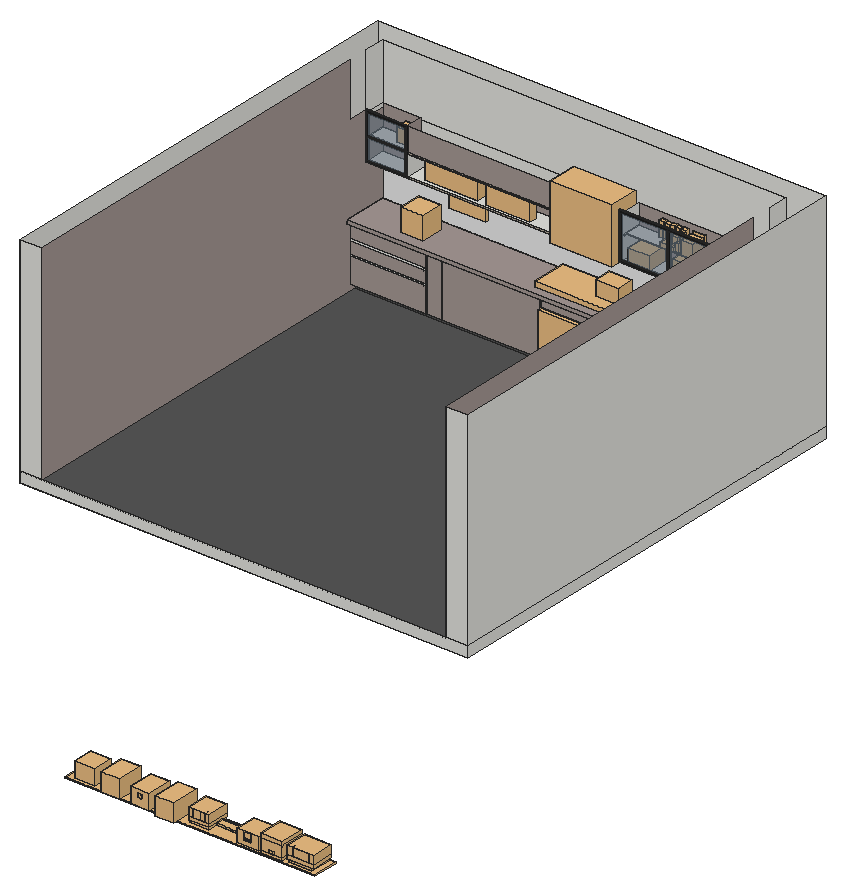
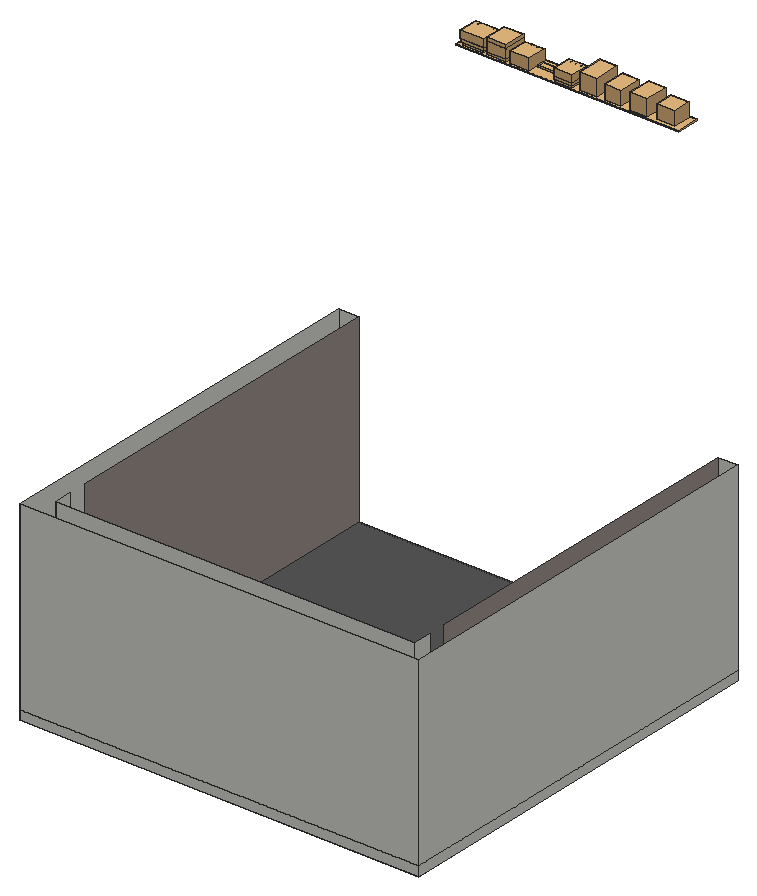
# SketchUp Ruby script. Lengths in inches.
U = 1.inch
M = Sketchup.active_model
def pt(a) = Geom::Point3d.new(a.map { |v| v * U })
def face(e, loops, mat)
  f = e.add_face(loops[0].map { |a| pt(a) })
  loops[1..].each { |l| e.add_face(l.map { |a| pt(a) }).erase! }
  f.material = f.back_material = mat if mat
  f
end
# faces: each face lists its corners as indices into pts; further lists are holes
def faces(e, pts, list, mat = nil) = list.each { |f| face(e, (f[0].is_a?(Array) ? f : [f]).map { |l| l.map { |i| pts[i] } }, mat) }
# xy, xz, yz: faces in a plane at the given z, y or x. An outline is a flat list of corners, or four numbers for a rectangle; further outlines are holes
def ring(l) = l.size == 4 ? [[l[0], l[1]], [l[2], l[1]], [l[2], l[3]], [l[0], l[3]]] : l.each_slice(2).to_a
def flat(e, list, mat, &to3) = list.each { |f| face(e, (f[0].is_a?(Array) ? f : [f]).map { |l| ring(l).map { |u, v| to3.(u, v) } }, mat) }
def xy(e, z, list, mat = nil) = flat(e, list, mat) { |x, y| [x, y, z] }
def xz(e, y, list, mat = nil) = flat(e, list, mat) { |x, z| [x, y, z] }
def yz(e, x, list, mat = nil) = flat(e, list, mat) { |y, z| [x, y, z] }
def lines(e, pts, list) = list.each { |a, b| e.add_line(pt(pts[a]), pt(pts[b])) }
# prism: a flat outline (further loops are holes) pulled along v
def prism(e, loops, v, mat = nil)
  f = face(e, loops, mat); d = Geom::Vector3d.new(v.map { |x| x * U })
  f.pushpull(f.normal.samedirection?(d) ? d.length : -d.length)
end
def box(e, o, s, mat = nil) = prism(e, [[o, [o[0] + s[0], o[1], o[2]], [o[0] + s[0], o[1] + s[1], o[2]], [o[0], o[1] + s[1], o[2]]]], [0, 0, s[2]], mat)
def at(x, y, z, deg = 0) = Geom::Transformation.translation(pt([x, y, z])) * Geom::Transformation.rotation(ORIGIN, Z_AXIS, deg.degrees)
def axes(o, x, y, z) = Geom::Transformation.new([*x, 0, *y, 0, *z, 0, *pt(o).to_a, 1])
def part(name) = M.definitions.add(name)
# library, detail: a bought-in or finely detailed component or shape, given as its bounding box
def library(name, o, s) = part(name).tap { |d| box(d.entities, o, s) }
def detail(e, o, s) = box(e.add_group.entities, o, s)
def put(e, d, t, mat = nil) = e.add_instance(d, t).tap { |i| i.material = mat if mat }
def group(e, t, mat = nil) = e.add_group.tap { |g| g.transformation = t; g.material = mat if mat }.entities
root = M.entities
M.materials.add("28").color = [48, 40, 35]
M.materials.add("29").color = [255, 248, 248]
M.materials.add("30").color = [174, 0, 0]
M.materials.add("7").color = [23, 21, 19]
M.materials.add("[0028_AntiqueWhite]").color = [183, 172, 157]
M.materials.add("[0110_LightSlateGray]").color = [119, 136, 153]
M.materials["[0110_LightSlateGray]"].alpha = 0.55
M.materials.add("[0132_LightGray]").color = [165, 152, 148]
M.materials.add("[Carpet Berber Pattern Gray]").color = [234, 234, 234]
M.materials.add("[Color M06]").color = [86, 86, 86]
M.materials.add("[Color M07]").color = [58, 58, 58]
M.materials.add("[Color M08]").color = [30, 30, 30]
c1 = library("Oven",[-9.26,-22.59,0.07],[23.42,23.91,23.21])
c2 = library("Sink with faucet",[0,-15.75,0],[23.62,20.08,14.64])
c3 = library("C_HOB",[0,0,0],[30.71,17.32,2.28])
c4 = library("wood+kitchen+tools (1)",[236.22,-4.93,0],[70.91,84.69,128.51])
c5 = library("hachoir 60",[0,0,0],[306.07,171.4,10.64])
c6 = part("hachoir année 60")
put(c6.entities,c5,at(-89.25,-74.89,-10.64))
c7 = library("Group\#91",[-0.04,-0.04,0],[12.83,12.7,13.07])
c8 = library("Lidded cooking pot",[0,0,0],[13.32,10.03,8.54])
c9 = library("skpC936",[0,-1.9,0],[21.12,3.04,12.85])
c10 = library("PV977NSS_GEProfile",[-17.9375,-27.5625,-0.25],[35.95,27.64,32.08])
c11 = library("Food+jars (2)",[-11.5,-3.52,0],[30.82,7.02,10])
c12 = library("jars",[-134.79,-4.32,0],[83.43,13.28,34.83])
c13 = library("Stocked cup rack",[0,0,0],[12.28,12.62,7.74])
c14 = library("Food+jars",[176.18,154.2,55.15],[6.14,23.65,7.76])
c15 = library("Stack of bowls \#1",[0,0,0],[8.98,8.99,10.96])
c16 = library("Group\#17",[-397.46,82.38,-0.11],[62.88,62.86,260])
c17 = library("Group\#16",[-282.65,82.375,-0.11],[62.85,62.875,260.02])
c18 = library("Group\#15",[222.96,189.98,-0.44],[259.48,39.25,337.49])
c19 = library("Group\#30",[41.52,-158.49,40.25],[95.93,90.14,172.87])
c20 = library("Group\#21",[-504.125,120.57,-0.1],[108.2,108.21,338.13])
c21 = library("Group\#22",[-376.9,120.94,-0.1],[107.79,107.8,326.37])
c22 = library("Group\#23",[-254.81,120.48,-0.6],[108.21,108.21,334.5])
c23 = library("Group\#24",[-133.01,121.19,-0.1],[106.95,106.95,324.89])
c24 = library("Group\#25",[0.46,121.12,-0.1],[106.94,106.94,338.14])
c25 = library("Group\#26",[151.35,137.54,-0.1],[70.51,70.14,256.45])
c26 = library("Group\#27",[-266.02,-201.27,40.23],[225.02,228.69,89.38])
c27 = library("Group\#28",[-78.56,-74.98,40.25],[131.28,107.59,245.3125])
c28 = library("Group\#31",[-60.55,-181.2,40.41],[105.85,106.35,65.49])
c29 = library("Group\#34",[253.59,42.68,151.97],[53.13,53.13,100.94])
c30 = library("Group\#35",[281.12,-5,151.97],[53.13,53.13,100.92])
c31 = library("Group\#36",[308.75,-52.85,151.97],[53.125,53.13,100.94])
c32 = library("Group\#37",[336.19,-100.38,151.98],[53.13,53.13,100.93])
c33 = library("Group\#38",[363.79,-148.1875,151.98],[53.13,53.13,100.93])
c34 = library("Group\#39",[253.59,42.68,30.7],[53.13,53.13,100.93])
c35 = library("Group\#40",[281.12,-5,30.7],[53.13,53.13,100.91])
c36 = library("Group\#41",[308.75,-52.85,30.7],[53.125,53.13,100.94])
c37 = library("Group\#42",[336.19,-100.38,30.7],[53.13,53.13,100.91])
c38 = library("Group\#43",[363.79,-148.1875,30.7],[53.13,53.13,100.93])
c39 = library("Group\#44",[212.54,-198.04,-0.24],[263.36,352.65,298.47])
c40 = library("Group\#29",[55.69,-19.19,40.37],[80.08,80.05,323.81])
c41 = part("KITCHEN+ITEMS+(1) (1)")
put(c41.entities,c16,at(0,0,0))
put(c41.entities,c17,at(0,0,0))
put(c41.entities,c18,at(0,0,0))
put(c41.entities,c19,at(0,0,-41.3))
put(c41.entities,c20,at(0,0,0))
put(c41.entities,c21,at(0,0,0))
put(c41.entities,c22,at(0,0,0))
put(c41.entities,c23,at(0,0,0))
put(c41.entities,c24,at(0,0,0))
put(c41.entities,c25,at(0,0,0))
put(c41.entities,c26,at(0,0,-41.3))
put(c41.entities,c27,at(0,0,-41.3))
put(c41.entities,c28,at(0,0,-41.3))
put(c41.entities,c29,at(0,0,0))
put(c41.entities,c30,at(0,0,0))
put(c41.entities,c31,at(0,0,0))
put(c41.entities,c32,at(0,0,0))
put(c41.entities,c33,at(0,0,0))
put(c41.entities,c34,at(0,0,0))
put(c41.entities,c35,at(0,0,0))
put(c41.entities,c36,at(0,0,0))
put(c41.entities,c37,at(0,0,0))
put(c41.entities,c38,at(0,0,0))
put(c41.entities,c39,at(0,0,0))
put(c41.entities,c40,at(0,0,-41.3))
c42 = library("Group58",[-1385.14,-3056.78,-20],[384.41,3679.22,19.83])
c43 = library("Group45",[-11.11,-120.87,-142.91],[286.39,35.1,309.1])
c44 = library("Group15",[-158.99,-158.99,-35.63],[317.98,317.98,183.08])
c45 = library("Group50",[-19.49,-140.71,-169.91],[291.24,11.25,339.82])
c46 = library("Group3",[-27.32,-120.87,-142.91],[318.81,35.07,309.1])
c47 = library("Group112",[-158.99,-158.99,-35.63],[317.98,317.98,245.51])
c48 = library("Group68",[-140.11,-219.43,-37.34],[282.52,424.43,265.46])
c49 = library("Group96",[-140.11,-174.24,-37.34],[282.52,379.24,265.46])
c50 = library("Group87",[-140.11,-176.26,-37.34],[282.52,381.26,230.21])
c51 = library("Group57",[-49.82,-129.46,-200.09],[351.89,311.64,400.18])
c52 = library("Group38",[-16.85,-85.77,-148.65],[297.88,51.33,320.95])
c53 = library("Group31",[-62.13,-16.41,-359.35],[127.68,33.17,391.44])
c54 = library("Group2",[-52.21,-87.55,-148.65],[368.59,53.1,320.95])
c55 = library("Group56",[-49.98,-85.16,-200.27],[352.22,199.23,400.54])
c56 = library("Group47",[-23.17,-23.17,1.84],[46.34,46.34,30.01])
c57 = library("Group25",[39913.82,7313.08,1428.86],[93.86,14.69,113.3])
c58 = part("om.cn_32940749")
prism(c58.entities,[[[-0.78,3.09,0],[0.53,4.43,0],[0.53,-4.51,0],[-0.78,-3.13,0]]],[0,0,1],"30")
c59 = part("om.cn_32112855")
prism(c59.entities,[[[-0.78,3.3125,0],[0.53,4.1875,0],[0.53,-4.32,0],[-0.78,-3.13,0]]],[0,0,1],"30")
c60 = part("om.cn_32889239")
xz(c60.entities,0,[[-3,0,3.22,1]],"30")
c61 = part("om.cn_3256117")
prism(c61.entities,[[[-3.59,0.4375,0],[3.59,0.4375,0],[3.68,0.43,0],[3.76,0.4,0],[3.84,0.35,0],[3.9,0.29,0],[3.94,0.21,0],[3.97,0.13,0],[3.98,0.04,0],[3.98,0.03,0],[3.97,-0.06,0],[3.94,-0.14,0],[3.9,-0.22,0],[3.84,-0.28,0],[3.76,-0.32,0],[3.68,-0.35,0],[3.59,-0.36,0],[-3.59,-0.36,0],[-3.68,-0.35,0],[-3.76,-0.32,0],[-3.84,-0.28,0],[-3.9,-0.22,0],[-3.94,-0.14,0],[-3.97,-0.06,0],[-3.98,0.03,0],[-3.98,0.04,0],[-3.97,0.13,0],[-3.94,0.21,0],[-3.9,0.29,0],[-3.84,0.35,0],[-3.76,0.4,0],[-3.68,0.43,0]]],[0,0,1],"29")
c62 = library("Group44",[-17.61,-34.44,-149.46],[299.39,113.28,322.55])
c63 = library("Group37",[-128.87,-80.45,-76.08],[259.72,160.9,77.15])
c64 = library("Group1",[-55.64,-34.64,-149.46],[375.46,113.48,322.55])
c65 = library("Group11",[40614.88,7323.5,1457.74],[233.16,50.23,111.04])
c66 = library("Group86",[38393.25,7253.08,1489.42],[61.25,2,52.13])
xy(root,-6,[[0,323.92,259.29,583.21]])
xy(root,0,[[0,323.92,12.74,323.92,12.74,550.47,246.55,550.47,246.55,323.92,259.29,323.92,259.29,583.21,0,583.21]])
xy(root,0,[[12.74,323.92,246.55,550.47]],"[Color M06]")
xy(root,4,[[12.74,546.47,12.74,550.47,246.55,550.47,246.55,546.47,217.72,546.47,217.72,546.78,217.42,546.78,217.42,546.47,188.6,546.47,188.6,546.78,188.3,546.78,188.3,546.47,160.91,546.47,160.91,546.78,160.61,546.78,160.61,546.47,123.66,546.47,123.66,546.78,123.36,546.78,123.36,546.47,66.6,546.47,66.6,546.78,66.3,546.78,66.3,546.47,57.35,546.47,57.35,546.78,57.05,546.78,57.05,546.47]])
xy(root,4.82,[[123.66,546.47,160.61,550.78],[123.66,550.78,160.61,573.03]])
xy(root,18.24,[[12.74,546.47,57.05,546.78]])
xy(root,19.61,[[12.74,546.47,57.05,546.78]])
xy(root,23.625,[[211.28,546.95,244.41,567.89]])
xy(root,26.07,[[12.74,546.47,57.05,546.78]])
xy(root,27.5,[[12.74,546.47,57.05,546.78]])
xy(root,30.22,[[123.66,546.47,160.61,550.78],[123.66,550.78,160.61,573.03]])
xy(root,36,[[12.74,544.47,12.74,546.47,57.05,546.47,57.05,546.78,57.35,546.78,57.35,546.47,66.3,546.47,66.3,546.78,66.6,546.78,66.6,546.47,123.36,546.47,123.36,546.78,123.66,546.78,123.66,546.47,160.61,546.47,160.61,546.78,160.91,546.78,160.91,546.47,188.3,546.47,188.3,546.78,188.6,546.78,188.6,546.47,217.42,546.47,217.42,546.78,217.72,546.78,217.72,546.47,246.55,546.47,246.55,544.47],[12.74,546.47,12.74,570.47,246.55,570.47,246.55,546.47,217.72,546.47,217.72,546.78,217.42,546.78,217.42,546.47,188.6,546.47,188.6,546.78,188.3,546.78,188.3,546.47,160.91,546.47,160.91,546.78,160.61,546.78,160.61,546.47,123.66,546.47,123.66,546.78,123.36,546.78,123.36,546.47,66.6,546.47,66.6,546.78,66.3,546.78,66.3,546.47,57.35,546.47,57.35,546.78,57.05,546.78,57.05,546.47]])
xy(root,38,[[[12.74,544.47,246.55,570.47],[211.28,546.95,244.41,567.89]]],"[0132_LightGray]")
xy(root,62,[[12.74,558.47,122.22,570.47],[160.125,558.47,246.55,570.47]])
xy(root,62.7,[[37.25,558.47,121.23,569.78]])
xy(root,62.98,[[13.72,558.47,35.57,569.78]])
xy(root,63.16,[[161.59,558.47,216.39,569.78]])
xy(root,74.79,[[13.72,560.41,35.57,569.78]])
xy(root,74.8,[[37.25,558.47,121.23,569.78]])
xy(root,75.5,[[13.72,560.41,35.57,569.78],[161.59,561.03,216.39,569.78]])
xy(root,76.36,[[161.59,561.03,216.39,569.78]])
xy(root,79.125,[[122.22,558.47,160.125,570.47]])
xz(root,323.92,[[0,-6,259.29,0],[0,0,12.74,120],[246.55,0,259.29,120]])
xz(root,544.47,[[12.74,36,246.55,38]],"[0132_LightGray]")
xz(root,546.47,[[123.66,4,160.61,4.82]])
xz(root,546.47,[[123.66,30.22,160.61,31.02]],"[0028_AntiqueWhite]")
xz(root,546.47,[[12.74,4,57.05,18.24],[57.35,4,66.3,36],[66.6,4,123.36,36],[160.91,4,188.3,36],[188.6,4,217.42,36],
  [217.72,4,246.55,36],[12.74,19.61,57.05,26.07],[12.74,27.5,57.05,36],[123.66,31.02,160.61,36]],"[0132_LightGray]")
xz(root,546.78,[[57.05,4,57.35,36],[66.3,4,66.6,36],[123.36,4,123.66,36],[160.61,4,160.91,36],[188.3,4,188.6,36],
  [217.42,4,217.72,36],[12.74,18.24,57.05,19.61],[12.74,26.07,57.05,27.5]])
xz(root,546.95,[[211.28,23.625,244.41,38]])
xz(root,550.47,[[12.74,0,246.55,4]],"[Color M06]")
xz(root,558.47,[[[12.74,62,36.55,89],[13.72,62.98,35.57,88.02]],[121.92,62,122.22,89],[160.125,62,160.42,89],[[160.42,62,217.55,89],[161.59,63.16,216.39,87.84]]])
xz(root,558.47,[[[36.55,62,121.92,75.5],[37.25,62.7,121.23,74.8]]],"[0028_AntiqueWhite]")
xz(root,558.47,[[217.55,62,246.55,89],[36.55,75.5,121.92,89],[122.22,79.125,160.125,89]],"[0132_LightGray]")
xz(root,560.41,[[13.72,74.79,35.57,75.5]])
xz(root,561.03,[[161.59,75.5,216.39,76.36]],"[0132_LightGray]")
xz(root,567.89,[[211.28,23.625,244.41,38]])
xz(root,569.78,[[13.72,74.79,35.57,75.5]])
xz(root,569.78,[[37.25,62.7,121.23,74.8],[13.72,62.98,35.57,74.79],[161.59,63.16,216.39,75.5],[13.72,75.5,35.57,88.02],[161.59,76.36,216.39,87.84]],"[0132_LightGray]")
xz(root,570.47,[[12.74,36,246.55,38],[12.74,62,12.74,86,246.55,86,246.55,62,160.125,62,160.125,79.125,122.22,79.125,122.22,62],[12.74,86,246.55,120]])
xz(root,570.47,[[12.74,38,246.55,62]],"[Carpet Berber Pattern Gray]")
xz(root,570.47,[[122.22,62,160.125,79.125]],"[Color M07]")
xz(root,573.03,[[123.66,4.82,160.61,30.22]])
xz(root,583.21,[[0,-6,259.29,0],[0,0,259.29,120]])
yz(root,0,[[323.92,-6,583.21,0],[323.92,0,583.21,120]])
yz(root,12.74,[[544.47,36,570.47,38],[558.47,62,570.47,86],[558.47,86,570.47,120]])
yz(root,12.74,[[323.92,0,550.47,0,550.47,4,546.47,4,546.47,18.24,546.78,18.24,546.78,19.61,546.47,19.61,546.47,26.07,546.78,26.07,546.78,27.5,546.47,27.5,546.47,36,544.47,36,544.47,38,570.47,38,570.47,62,558.47,62,558.47,89,546.47,89,546.47,120,323.92,120]],"[0132_LightGray]")
yz(root,13.72,[[558.47,74.79,560.41,75.5],[560.41,74.79,569.78,75.5],[558.47,86,569.78,88.02]])
yz(root,13.72,[[558.47,62.98,569.78,74.79],[558.47,75.5,569.78,86]],"[0132_LightGray]")
yz(root,35.57,[[558.47,74.79,560.41,75.5],[560.41,74.79,569.78,75.5]])
yz(root,35.57,[[558.47,62.98,569.78,74.79],[558.47,75.5,569.78,88.02]],"[0132_LightGray]")
yz(root,37.25,[[558.47,62.7,569.78,74.8]])
yz(root,57.05,[[546.47,4,546.78,18.24],[546.47,19.61,546.78,26.07],[546.47,27.5,546.78,36]])
yz(root,57.35,[[546.47,4,546.78,36]])
yz(root,66.3,[[546.47,4,546.78,36]])
yz(root,66.6,[[546.47,4,546.78,36]])
yz(root,121.23,[[558.47,62.7,569.78,74.8]])
yz(root,122.22,[[558.47,62,570.47,79.125]])
yz(root,123.36,[[546.47,4,546.78,36]])
yz(root,123.66,[[546.47,4,546.78,4.82],[546.78,4.82,550.78,30.22],[550.78,4.82,573.03,30.22],[546.47,30.22,546.78,36]])
yz(root,160.125,[[558.47,62,570.47,79.125]])
yz(root,160.61,[[546.47,4,546.78,4.82],[546.78,4.82,550.78,30.22],[550.78,4.82,573.03,30.22],[546.47,30.22,546.78,36]])
yz(root,160.91,[[546.47,4,546.78,36]])
yz(root,161.59,[[558.47,63.16,569.78,63.16,569.78,75.25,559.1,75.25,559.1,75.5,558.47,75.5],[559.1,75.25,569.78,75.5],[558.47,75.5,561.03,76.36],[561.03,75.5,569.78,76.36],[558.47,76.36,569.78,87.84]])
yz(root,188.3,[[546.47,4,546.78,36]])
yz(root,188.6,[[546.47,4,546.78,36]])
yz(root,211.28,[[546.95,23.625,567.89,38]])
yz(root,216.39,[[558.47,75.5,561.03,76.36]])
yz(root,216.39,[[558.47,63.16,569.78,75.5],[558.47,76.36,569.78,87.84]],"[0132_LightGray]")
yz(root,217.42,[[546.47,4,546.78,36]])
yz(root,217.72,[[546.47,4,546.78,36]])
yz(root,244.41,[[546.95,23.625,567.89,38]])
yz(root,246.55,[[544.47,36,570.47,38],[558.47,62,570.47,86],[558.47,86,570.47,120]])
yz(root,246.55,[[323.92,0,323.92,120,546.47,120,546.47,89,558.47,89,558.47,62,570.47,62,570.47,38,544.47,38,544.47,36,546.47,36,546.47,4,550.47,4,550.47,0]],"[0132_LightGray]")
yz(root,259.29,[[323.92,-6,583.21,0],[323.92,0,583.21,120]])
put(root,c1,axes([138.2,566.93,4.68],[1.57,0,0],[0,1,0],[0,0,1.09434]))
put(root,c2,axes([211.47,565.41,33.375],[1.41,0,0],[0,1.16965,0],[0,0,1]))
put(root,c3,axes([117.7,549.54,38],[1.4986,0,0],[0,1.18,0],[0,0,1.18]))
put(root,c4,axes([175.76,559.98,38],[0.0693,0,0],[0,0.0693,0],[0,0,0.0693]))
put(root,c6,axes([196.83,568.68,48.68],[0,0,-0.04924],[0.062,0,0],[0,-0.062,0]))
put(root,c7,at(39.22,551.01,38))
put(root,c8,at(147.64,556.12,40.62))
put(root,c9,at(52.79,570.47,47.72))
put(root,c10,at(141.68,580.64,61.58))
g1 = group(root,at(160.125,557.41,62),"[Color M08]")
xy(g1,0,[[0,0,57.125,1.0625]])
xy(g1,1.16,[[1.16,0,27.91,0.53],[27.91,0,28.5625,1.0625],[28.5625,0,29.22,1.0625],[29.22,0,55.96,0.53],[1.16,0.53,27.91,1.0625],
  [29.22,0.53,55.96,1.0625]])
xy(g1,25.84,[[1.16,0,27.91,0.53],[27.91,0,28.5625,1.0625],[29.22,0,55.96,0.53],[1.16,0.53,27.91,1.0625],[29.22,0.53,55.96,1.0625]])
xy(g1,27,[[0,0,57.125,1.0625]])
xz(g1,0,[[[0,0,57.125,27],[1.16,1.16,55.96,25.84]],[27.91,1.16,28.5625,25.84],[28.5625,1.16,29.22,25.84]])
xz(g1,0.53,[[1.16,1.16,27.91,25.84],[29.22,1.16,55.96,25.84]],"[0110_LightSlateGray]")
xz(g1,1.0625,[[[0,0,57.125,27],[1.16,1.16,55.96,25.84]],[27.91,1.16,28.5625,25.84],[28.5625,1.16,29.22,25.84]])
yz(g1,0,[[0,0,1.0625,27]])
yz(g1,1.16,[[0,1.16,0.53,25.84],[0.53,1.16,1.0625,25.84]])
yz(g1,27.91,[[0,1.16,0.53,25.84],[0.53,1.16,1.0625,25.84]])
yz(g1,28.5625,[[0,1.16,1.0625,25.84]])
yz(g1,29.22,[[0,1.16,0.53,25.84],[0.53,1.16,1.0625,25.84]])
yz(g1,55.96,[[0,1.16,0.53,25.84],[0.53,1.16,1.0625,25.84]])
yz(g1,57.125,[[0,0,1.0625,27]])
g2 = group(root,at(13.33,557.47,62.36),"[Color M08]")
xy(g2,0,[[0,0,23.8125,1]])
xy(g2,0.98,[[0.98,0,22.83,0.5],[0.98,0.5,22.83,1]])
xy(g2,13.07,[[0.98,0,22.83,0.5],[0.98,0.5,22.83,1]])
xy(g2,13.5,[[0.98,0,22.83,1]])
xy(g2,13.9,[[0.98,0,22.83,0.5],[0.98,0.5,22.83,1]])
xy(g2,26.02,[[0.98,0,22.83,0.5],[0.98,0.5,22.83,1]])
xy(g2,27,[[0,0,23.8125,1]])
xz(g2,0,[[[0,0,23.8125,27],[0.98,0.98,22.83,26.02]],[0.98,13.07,22.83,13.5],[0.98,13.5,22.83,13.9]])
xz(g2,0.5,[[0.98,0.98,22.83,13.07],[0.98,13.9,22.83,26.02]],"[0110_LightSlateGray]")
xz(g2,1,[[[0,0,23.8125,27],[0.98,0.98,22.83,26.02]],[0.98,13.07,22.83,13.5],[0.98,13.5,22.83,13.9]])
yz(g2,0,[[0,0,1,24],[0,24,1,27]])
yz(g2,0.98,[[0,0.98,0.5,13.07],[0.5,0.98,1,13.07],[0,13.07,1,13.5],[0,13.5,1,13.9],[0,13.9,0.5,26.02],
  [0.5,13.9,1,26.02]])
yz(g2,22.83,[[0,0.98,0.5,13.07],[0.5,0.98,1,13.07],[0,13.5,1,13.9],[0,13.9,0.5,26.02],[0.5,13.9,1,26.02]])
yz(g2,23.8125,[[0,0,1,13.5],[0,13.5,1,27]])
put(root,c11,at(56.02,564.64,62.7))
put(root,c12,axes([122.43,561.67,62.7],[0.3105,0,0],[0,0.3105,0],[0,0,0.3105]))
put(root,c13,at(164.8,558.47,63.16))
put(root,c14,at(32.79,744.86,8.02,-90))
put(root,c15,axes([27.16,562.93,75.5],[0.72,0,0],[0,0.72,0],[0,0,0.72]))
put(root,c41,axes([188.29,564.8,76.38],[0.0253,0,0],[0,0.02176,0],[0,0,0.0253]))
put(root,c42,axes([403.23,-36.38,80.58],[0,-0.03937,0],[0.03937,0,0],[0,0,-0.03937]))
put(root,c43,axes([353.2,12.12,86.11],[0.03937,0,0],[0,0,0.03937],[0,-0.03937,0]))
put(root,c44,axes([387.39,10.73,82.75],[0.03937,0,0],[0,0.03937,0],[0,0,0.03937]))
put(root,c45,axes([397.57,10.42,85.8],[0.03558,0,0],[0,0,0.03166],[0,-0.03558,0]))
put(root,c46,axes([412.2,11.58,86.46],[0.0415,0,0],[0,0,0.0415],[0,-0.03937,0]))
put(root,c47,axes([292.91,10.24,82.88],[0.03687,0,0],[0,0.03687,0],[0,0,0.03687]))
put(root,c48,axes([342.84,8.64,83.09],[0.03937,0,0],[0,0.03937,0],[0,0,0.03937]))
put(root,c49,axes([309.68,8.95,83.09],[0.03937,0,0],[0,0.03937,0],[0,0,0.03937]))
put(root,c50,axes([326.82,8.82,83.09],[0.03862,0,0],[0,0.03862,0],[0,0,0.03862]))
put(root,c51,axes([397.57,10.42,85.8],[0.03558,0,0],[0,0,0.03166],[0,-0.03558,0]))
put(root,c52,axes([353.2,12.12,86.11],[0.03937,0,0],[0,0,0.03937],[0,-0.03937,0]))
put(root,c53,axes([366.625,11.35,83.29],[-0.00028,-0.03231,0],[0,0,0.03231],[-0.03231,0.00028,0]))
put(root,c54,axes([412.2,11.61,86.5],[0.0415,0,0],[0,0,0.0415],[0,-0.03937,0]))
put(root,c55,axes([397.57,10.42,85.8],[0.03558,0,0],[0,0,0.03166],[0,-0.03558,0]))
g3 = group(root,at(397.57,10.42,85.8))
p = [[3.89,-6.65,3.07],[3.11,-6.99,-2.16],[3.79,-7.09,-2.57],[3.79,-7.06,-2.16],[3.09,-7.02,-2.57],[4.49,-7.12,-2.57],
  [4.49,-6.67,3.07],[5.19,-7.09,-2.57],[5.18,-7.06,-2.16],[5.09,-6.65,3.07],[5.87,-6.99,-2.16],[5.88,-7.02,-2.57],
  [2.4375,-6.88,-2.16],[2.42,-6.92,-2.57],[6.54,-6.88,-2.16],[6.56,-6.92,-2.57],[1.79,-6.74,-2.16],[1.77,-6.77,-2.57],
  [7.18,-6.74,-2.16],[7.21,-6.77,-2.57],[1.18,-6.57,-2.16],[1.15,-6.59,-2.57],[7.8,-6.57,-2.16],[7.83,-6.59,-2.57],
  [0.61,-6.35,-2.16],[0.58,-6.375,-2.57],[8.37,-6.35,-2.16],[8.4,-6.375,-2.57],[0.1,-6.07,-2.16],[0.07,-6.1,-2.57],
  [8.88,-6.07,-2.16],[8.91,-6.1,-2.57],[-0.12,-5.95,-2.5],[9.09,-5.95,-2.5],[-0.27,-5.8125,-2.33],[0.47,-5.7,3.07],
  [0.13,-5.41,3.24],[0.05,-5.375,3.07],[-0.32,-5.75,-2.15],[9.24,-5.8125,-2.33],[9.3,-5.75,-2.15],[8.92,-5.375,3.07],
  [8.84,-5.41,3.24],[8.51,-5.7,3.07],[4.49,-6.64,3.48],[3.9,-6.62,3.48],[5.08,-6.62,3.48],[2.7,-6.49,3.07],
  [3.29,-6.59,3.07],[3.31,-6.5625,3.48],[5.6875,-6.59,3.07],[5.67,-6.5625,3.48],[6.28,-6.49,3.07],[2.11,-6.36,3.07],
  [6.87,-6.36,3.07],[1.53,-6.1875,3.07],[7.44,-6.1875,3.07],[0.98,-5.97,3.07],[8,-5.97,3.07],[2.72,-6.46,3.48],
  [6.26,-6.46,3.48],[2.14,-6.33,3.48],[6.84,-6.33,3.48],[1.56,-6.16,3.48],[7.42,-6.16,3.48],[1.01,-5.94,3.48],
  [7.97,-5.94,3.48],[0.51,-5.67,3.48],[8.47,-5.67,3.48],[0.3125,-5.53,3.41],[8.66,-5.53,3.41]]
faces(g3,p,[[0,1,2,3],[1,4,2],[2,5,6,3],[6,5,7,8],[9,8,7,10],[7,11,10],[12,13,4],[4,1,12],
  [14,10,11],[11,15,14],[16,17,13],[13,12,16],[18,14,15],[15,19,18],[20,21,17],[17,16,20],
  [22,18,19],[19,23,22],[24,25,21],[21,20,24],[26,22,23],[23,27,26],[28,29,25],[25,24,28],
  [30,26,27],[27,31,30],[32,29,28],[30,31,33],[34,32,28,35,36,37,38],[30,33,39,40,41,42,43],[44,45,0,3,6],[9,46,44,6,8],
  [47,12,1],[1,48,47],[1,0,49,48],[10,50,51,9],[52,50,10],[10,14,52],[53,16,12],[12,47,53],
  [54,52,14],[14,18,54],[55,20,16],[16,53,55],[56,54,18],[18,22,56],[57,24,20],[20,55,57],
  [58,56,22],[22,26,58],[28,24,57],[58,26,30],[57,35,28],[30,43,58],[0,45,49],[51,46,9],
  [48,49,59],[59,47,48],[50,52,60],[60,51,50],[47,59,61],[61,53,47],[52,54,62],[62,60,52],
  [63,55,53],[53,61,63],[64,62,54],[54,56,64],[55,63,65],[65,57,55],[56,58,66],[66,64,56],
  [57,65,67],[67,35,57],[58,43,68],[68,66,58],[69,36,35,67],[70,68,43,42]],"7")
put(root,c56,axes([402.0625,3.97,84.18],[-0.05506,0,0],[0,0,0.03202],[0,-0.03202,0]))
put(root,c57,axes([-1185.85,-283.55,27.72],[0.03937,0,0],[0,0.03937,0],[0,0,0.03937]))
put(root,c58,axes([387.43,4.36,84.54],[0,-0.00453,-0.03911],[-0.03514,0,0],[0,-0.03911,0.00453]))
put(root,c59,axes([387.58,4.375,84.71],[0.03514,0,0],[0,0.00453,0.03911],[0,-0.03911,0.00453]))
put(root,c59,axes([387.28,4.375,84.71],[-0.03514,0,0],[0,0.00453,0.03911],[0,-0.03911,0.00453]))
put(root,c60,axes([387.42,4.36,84.57],[0.03514,0,0],[0,0.00453,0.03911],[0,-0.03911,0.00453]))
put(root,c61,axes([388.6,4.39,84.86],[0,-0.00453,-0.03911],[0.03514,0,0],[0,-0.02541,0.00294]))
put(root,c62,axes([353.2,12.12,86.11],[0.03937,0,0],[0,0,0.03937],[0,-0.03937,0]))
put(root,c63,axes([358.41,5.34,86.91],[0.02601,-0.00023,0],[0,0,0.02576],[-0.00023,-0.02601,0]))
put(root,c61,axes([388.6,4.39,84.86],[0.03514,0,0],[0,0.00453,0.03911],[0,-0.03911,0.00453]))
put(root,c61,axes([386.24,4.39,84.875],[0.03514,0,0],[0,0.00453,0.03911],[0,-0.03911,0.00453]))
put(root,c60,axes([387.42,4.39,84.86],[0.03514,0,0],[0,-0.00453,-0.03911],[0,-0.03911,0.00453]))
put(root,c58,axes([387.43,4.4,84.89],[0,0.00453,0.03911],[-0.03514,0,0],[0,-0.03911,0.00453]))
put(root,c59,axes([387.28,4.42,85.08],[-0.03514,0,0],[0,0.00453,0.03911],[0,-0.03911,0.00453]))
put(root,c64,axes([412.2,11.61,86.5],[0.0415,0,0],[0,0,0.0415],[0,-0.03937,0]))
put(root,c65,axes([-1185.85,-283.55,27.72],[0.03937,0,0],[0,0.03937,0],[0,0,0.03937]))
g4 = group(root,at(-1185.85,-283.55,27.72))
xz(g4,287.93,[[1571.78,57.46,1574.74,57.46,1571.73,57.47],[1574.74,57.46,1574.78,57.47,1574.81,57.48],[1574.81,57.48,1574.83,57.49,1574.85,57.52],[1571.6875,57.49,1571.65,57.54,1571.67,57.52],[1574.85,57.52,1574.86,57.54,1574.87,57.57]],"28")
p = [[1574.87,287.93,57.57],[1574.875,288.09,60.4],[1571.64,288.09,60.4],[1571.64,287.93,57.62],[1571.64,287.93,57.57],[1571.65,287.93,57.54],
  [1571.6875,287.93,57.49],[1571.71,287.93,57.48],[1571.73,287.93,57.47],[1574.74,287.93,57.46],[1574.81,287.93,57.48],[1574.85,287.93,57.52],
  [1574.875,287.93,57.62]]
faces(g4,p,[[0,1,2,3,4,5,6,7,8,9,10,11],[0,12,1]],"28")
put(root,c66,axes([-1185.85,-283.55,27.72],[0.03937,0,0],[0,0.03937,0],[0,0,0.03937]))
